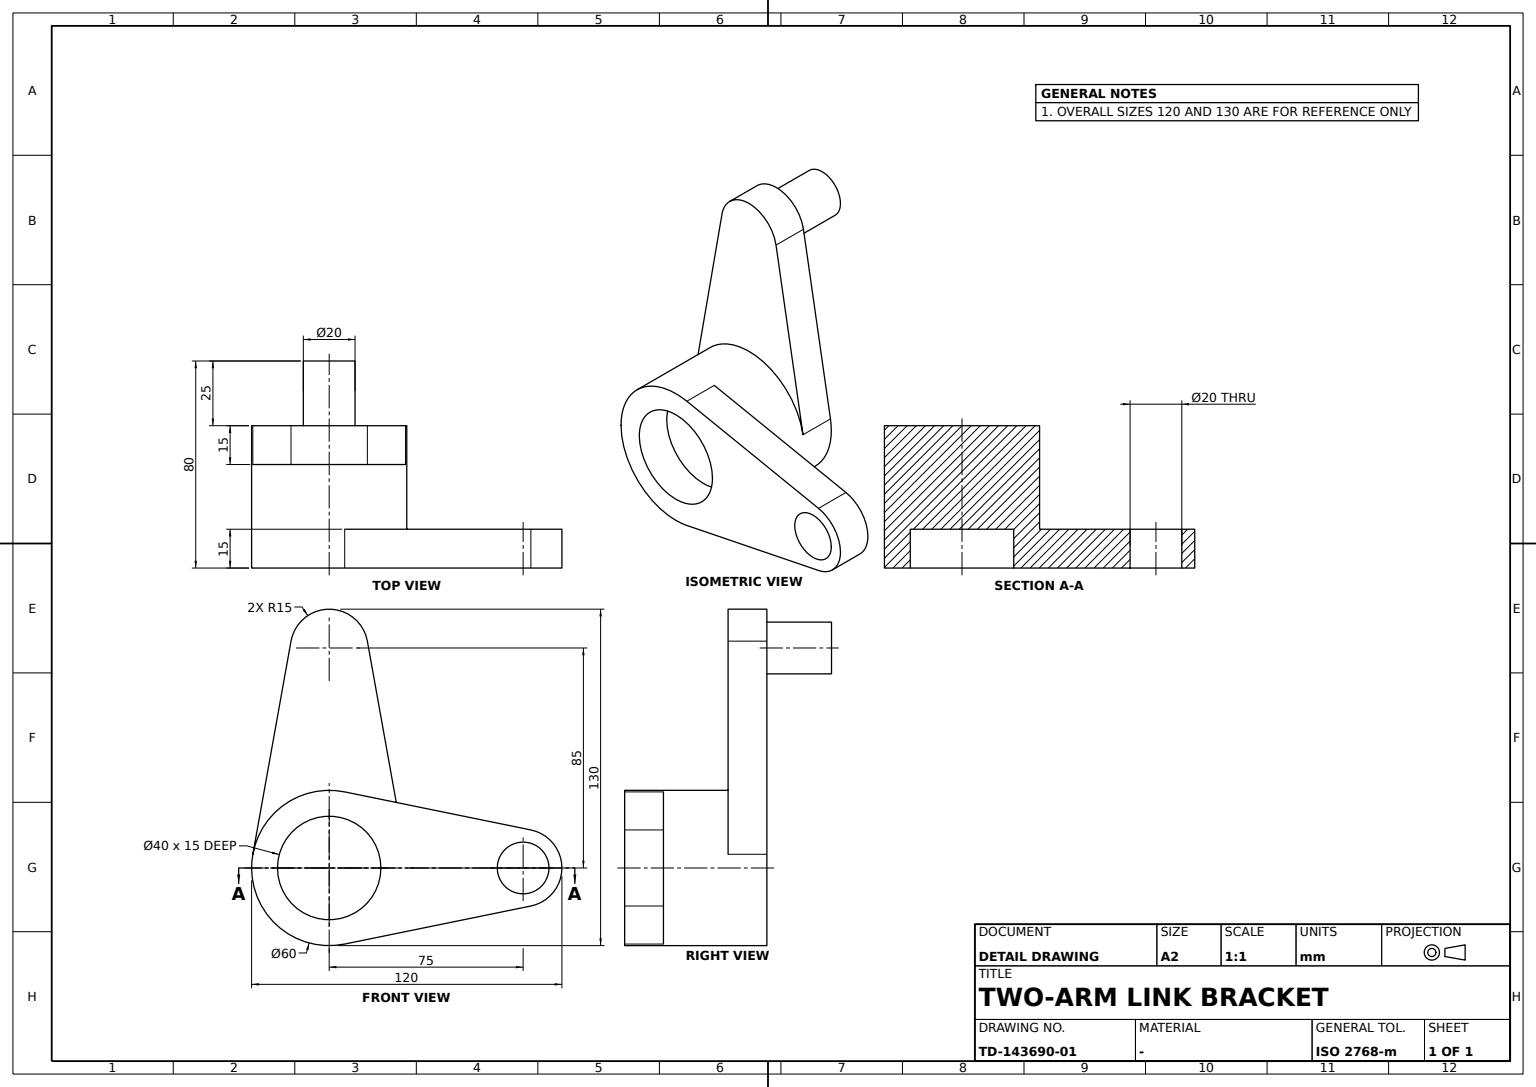
ISO-10303-21;
HEADER;
FILE_DESCRIPTION((''),'2;1');
FILE_NAME('','',(''),(''),'','','');
FILE_SCHEMA(('AUTOMOTIVE_DESIGN'));
ENDSEC;
DATA;
#1=APPLICATION_CONTEXT('');
#2=PRODUCT_CONTEXT('',#1,'mechanical');
#3=PRODUCT('','','',(#2));
#4=PRODUCT_DEFINITION_FORMATION('','',#3);
#5=PRODUCT_DEFINITION_CONTEXT('',#1,'design');
#6=PRODUCT_DEFINITION('','',#4,#5);
#7=PRODUCT_DEFINITION_SHAPE('','',#6);
#8=(LENGTH_UNIT()NAMED_UNIT(*)SI_UNIT(.MILLI.,.METRE.));
#9=(NAMED_UNIT(*)PLANE_ANGLE_UNIT()SI_UNIT($,.RADIAN.));
#10=(NAMED_UNIT(*)SI_UNIT($,.STERADIAN.)SOLID_ANGLE_UNIT());
#11=UNCERTAINTY_MEASURE_WITH_UNIT(LENGTH_MEASURE(1.E-05),#8,'distance_accuracy_value','');
#12=(GEOMETRIC_REPRESENTATION_CONTEXT(3)GLOBAL_UNCERTAINTY_ASSIGNED_CONTEXT((#11))GLOBAL_UNIT_ASSIGNED_CONTEXT((#8,#9,#10))REPRESENTATION_CONTEXT('',''));
#13=CARTESIAN_POINT('',(40.,85.,0.));
#14=VERTEX_POINT('',#13);
#15=CARTESIAN_POINT('',(40.,65.,0.));
#16=VERTEX_POINT('',#15);
#17=CARTESIAN_POINT('',(40.,75.,0.));
#18=DIRECTION('',(1.,0.,0.));
#19=DIRECTION('',(0.,1.,0.));
#20=AXIS2_PLACEMENT_3D('',#17,#18,#19);
#21=CIRCLE('',#20,10.);
#22=EDGE_CURVE('',#14,#16,#21,.T.);
#23=ORIENTED_EDGE('',*,*,#22,.F.);
#24=CARTESIAN_POINT('',(55.,85.,0.));
#25=VERTEX_POINT('',#24);
#26=CARTESIAN_POINT('',(47.5,85.,0.));
#27=DIRECTION('',(-1.,0.,0.));
#28=VECTOR('',#27,1000.);
#29=LINE('',#26,#28);
#30=EDGE_CURVE('',#25,#14,#29,.T.);
#31=ORIENTED_EDGE('',*,*,#30,.F.);
#32=CARTESIAN_POINT('',(55.,65.,0.));
#33=VERTEX_POINT('',#32);
#34=CARTESIAN_POINT('',(55.,75.,0.));
#35=AXIS2_PLACEMENT_3D('',#34,#18,#19);
#36=CIRCLE('',#35,10.);
#37=EDGE_CURVE('',#25,#33,#36,.T.);
#38=ORIENTED_EDGE('',*,*,#37,.T.);
#39=CARTESIAN_POINT('',(47.5,65.,0.));
#40=LINE('',#39,#28);
#41=EDGE_CURVE('',#33,#16,#40,.T.);
#42=ORIENTED_EDGE('',*,*,#41,.T.);
#43=EDGE_LOOP('',(#23,#31,#38,#42));
#44=FACE_OUTER_BOUND('',#43,.T.);
#45=CARTESIAN_POINT('',(47.5,75.,0.));
#46=AXIS2_PLACEMENT_3D('',#45,#27,#19);
#47=CYLINDRICAL_SURFACE('',#46,10.);
#48=ADVANCED_FACE('',(#44),#47,.F.);
#49=CARTESIAN_POINT('',(0.,-10.,85.));
#50=VERTEX_POINT('',#49);
#51=CARTESIAN_POINT('',(0.,10.,85.));
#52=VERTEX_POINT('',#51);
#53=CARTESIAN_POINT('',(0.,0.,85.));
#54=DIRECTION('',(0.,-1.,0.));
#55=AXIS2_PLACEMENT_3D('',#53,#27,#54);
#56=CIRCLE('',#55,10.);
#57=EDGE_CURVE('',#50,#52,#56,.T.);
#58=ORIENTED_EDGE('',*,*,#57,.F.);
#59=EDGE_CURVE('',#52,#50,#56,.T.);
#60=ORIENTED_EDGE('',*,*,#59,.F.);
#61=EDGE_LOOP('',(#58,#60));
#62=FACE_BOUND('',#61,.T.);
#63=CARTESIAN_POINT('',(0.,-14.764587,87.64707));
#64=VERTEX_POINT('',#63);
#65=CARTESIAN_POINT('',(0.,-29.529175,5.294128));
#66=VERTEX_POINT('',#65);
#67=CARTESIAN_POINT('',(0.,-22.146881,46.470599));
#68=DIRECTION('',(0.,-0.176470588,-0.984305914));
#69=VECTOR('',#68,1000.);
#70=LINE('',#67,#69);
#71=EDGE_CURVE('',#64,#66,#70,.T.);
#72=ORIENTED_EDGE('',*,*,#71,.F.);
#73=CARTESIAN_POINT('',(0.,14.764589,87.647059));
#74=VERTEX_POINT('',#73);
#75=AXIS2_PLACEMENT_3D('',#53,#18,#19);
#76=CIRCLE('',#75,15.);
#77=EDGE_CURVE('',#74,#64,#76,.T.);
#78=ORIENTED_EDGE('',*,*,#77,.F.);
#79=CARTESIAN_POINT('',(0.,29.529177,5.294118));
#80=VERTEX_POINT('',#79);
#81=CARTESIAN_POINT('',(0.,22.146883,46.470588));
#82=DIRECTION('',(0.,0.176470588,-0.984305914));
#83=VECTOR('',#82,1000.);
#84=LINE('',#81,#83);
#85=EDGE_CURVE('',#74,#80,#84,.T.);
#86=ORIENTED_EDGE('',*,*,#85,.T.);
#87=CARTESIAN_POINT('',(0.,30.,0.));
#88=VERTEX_POINT('',#87);
#89=CARTESIAN_POINT('',(0.,0.,0.));
#90=AXIS2_PLACEMENT_3D('',#89,#18,#19);
#91=CIRCLE('',#90,30.);
#92=EDGE_CURVE('',#88,#80,#91,.T.);
#93=ORIENTED_EDGE('',*,*,#92,.F.);
#94=CARTESIAN_POINT('',(0.,-30.,0.));
#95=VERTEX_POINT('',#94);
#96=EDGE_CURVE('',#95,#88,#91,.T.);
#97=ORIENTED_EDGE('',*,*,#96,.F.);
#98=EDGE_CURVE('',#66,#95,#91,.T.);
#99=ORIENTED_EDGE('',*,*,#98,.F.);
#100=EDGE_LOOP('',(#72,#78,#86,#93,#97,#99));
#101=FACE_OUTER_BOUND('',#100,.T.);
#102=PLANE('',#90);
#103=ADVANCED_FACE('',(#62,#101),#102,.F.);
#104=EDGE_CURVE('',#33,#25,#36,.T.);
#105=ORIENTED_EDGE('',*,*,#104,.T.);
#106=ORIENTED_EDGE('',*,*,#30,.T.);
#107=EDGE_CURVE('',#16,#14,#21,.T.);
#108=ORIENTED_EDGE('',*,*,#107,.F.);
#109=ORIENTED_EDGE('',*,*,#41,.F.);
#110=EDGE_LOOP('',(#105,#106,#108,#109));
#111=FACE_OUTER_BOUND('',#110,.T.);
#112=ADVANCED_FACE('',(#111),#47,.F.);
#113=CARTESIAN_POINT('',(40.,78.,-14.696938));
#114=VERTEX_POINT('',#113);
#115=CARTESIAN_POINT('',(40.,90.,0.));
#116=VERTEX_POINT('',#115);
#117=CIRCLE('',#20,15.);
#118=EDGE_CURVE('',#114,#116,#117,.T.);
#119=ORIENTED_EDGE('',*,*,#118,.T.);
#120=CARTESIAN_POINT('',(55.,90.,0.));
#121=VERTEX_POINT('',#120);
#122=CARTESIAN_POINT('',(47.5,90.,0.));
#123=LINE('',#122,#28);
#124=EDGE_CURVE('',#121,#116,#123,.T.);
#125=ORIENTED_EDGE('',*,*,#124,.F.);
#126=CARTESIAN_POINT('',(55.,78.,-14.696938));
#127=VERTEX_POINT('',#126);
#128=CIRCLE('',#35,15.);
#129=EDGE_CURVE('',#127,#121,#128,.T.);
#130=ORIENTED_EDGE('',*,*,#129,.F.);
#131=CARTESIAN_POINT('',(47.5,78.,-14.696938));
#132=LINE('',#131,#28);
#133=EDGE_CURVE('',#127,#114,#132,.T.);
#134=ORIENTED_EDGE('',*,*,#133,.T.);
#135=EDGE_LOOP('',(#119,#125,#130,#134));
#136=FACE_OUTER_BOUND('',#135,.T.);
#137=CYLINDRICAL_SURFACE('',#46,15.);
#138=ADVANCED_FACE('',(#136),#137,.T.);
#139=CARTESIAN_POINT('',(-25.,10.,85.));
#140=VERTEX_POINT('',#139);
#141=CARTESIAN_POINT('',(-12.5,10.,85.));
#142=LINE('',#141,#28);
#143=EDGE_CURVE('',#52,#140,#142,.T.);
#144=ORIENTED_EDGE('',*,*,#143,.F.);
#145=ORIENTED_EDGE('',*,*,#59,.T.);
#146=CARTESIAN_POINT('',(-25.,-10.,85.));
#147=VERTEX_POINT('',#146);
#148=CARTESIAN_POINT('',(-12.5,-10.,85.));
#149=LINE('',#148,#28);
#150=EDGE_CURVE('',#50,#147,#149,.T.);
#151=ORIENTED_EDGE('',*,*,#150,.T.);
#152=CARTESIAN_POINT('',(-25.,0.,85.));
#153=AXIS2_PLACEMENT_3D('',#152,#27,#54);
#154=CIRCLE('',#153,10.);
#155=EDGE_CURVE('',#140,#147,#154,.T.);
#156=ORIENTED_EDGE('',*,*,#155,.F.);
#157=EDGE_LOOP('',(#144,#145,#151,#156));
#158=FACE_OUTER_BOUND('',#157,.T.);
#159=CARTESIAN_POINT('',(-12.5,0.,85.));
#160=AXIS2_PLACEMENT_3D('',#159,#18,#54);
#161=CYLINDRICAL_SURFACE('',#160,10.);
#162=ADVANCED_FACE('',(#158),#161,.T.);
#163=CARTESIAN_POINT('',(40.,78.,14.696938));
#164=VERTEX_POINT('',#163);
#165=CARTESIAN_POINT('',(40.,6.,29.393877));
#166=VERTEX_POINT('',#165);
#167=CARTESIAN_POINT('',(40.,42.,22.045408));
#168=DIRECTION('',(0.,-0.979795897,0.2));
#169=VECTOR('',#168,1000.);
#170=LINE('',#167,#169);
#171=EDGE_CURVE('',#164,#166,#170,.T.);
#172=ORIENTED_EDGE('',*,*,#171,.F.);
#173=EDGE_CURVE('',#116,#164,#117,.T.);
#174=ORIENTED_EDGE('',*,*,#173,.F.);
#175=ORIENTED_EDGE('',*,*,#118,.F.);
#176=CARTESIAN_POINT('',(40.,6.,-29.393877));
#177=VERTEX_POINT('',#176);
#178=CARTESIAN_POINT('',(40.,42.,-22.045408));
#179=DIRECTION('',(0.,0.979795897,0.2));
#180=VECTOR('',#179,1000.);
#181=LINE('',#178,#180);
#182=EDGE_CURVE('',#177,#114,#181,.T.);
#183=ORIENTED_EDGE('',*,*,#182,.F.);
#184=CARTESIAN_POINT('',(40.,30.,0.));
#185=VERTEX_POINT('',#184);
#186=CARTESIAN_POINT('',(40.,0.,0.));
#187=AXIS2_PLACEMENT_3D('',#186,#18,#19);
#188=CIRCLE('',#187,30.);
#189=EDGE_CURVE('',#177,#185,#188,.T.);
#190=ORIENTED_EDGE('',*,*,#189,.T.);
#191=CARTESIAN_POINT('',(40.,29.529177,5.294118));
#192=VERTEX_POINT('',#191);
#193=EDGE_CURVE('',#185,#192,#188,.T.);
#194=ORIENTED_EDGE('',*,*,#193,.T.);
#195=AXIS2_PLACEMENT_3D('',#186,#27,#19);
#196=CIRCLE('',#195,30.);
#197=EDGE_CURVE('',#166,#192,#196,.T.);
#198=ORIENTED_EDGE('',*,*,#197,.F.);
#199=EDGE_LOOP('',(#172,#174,#175,#183,#190,#194,#198));
#200=FACE_OUTER_BOUND('',#199,.T.);
#201=ORIENTED_EDGE('',*,*,#107,.T.);
#202=ORIENTED_EDGE('',*,*,#22,.T.);
#203=EDGE_LOOP('',(#201,#202));
#204=FACE_BOUND('',#203,.T.);
#205=PLANE('',#187);
#206=ADVANCED_FACE('',(#200,#204),#205,.F.);
#207=CARTESIAN_POINT('',(40.,-20.,0.));
#208=VERTEX_POINT('',#207);
#209=CARTESIAN_POINT('',(40.,20.,0.));
#210=VERTEX_POINT('',#209);
#211=CIRCLE('',#187,20.);
#212=EDGE_CURVE('',#208,#210,#211,.T.);
#213=ORIENTED_EDGE('',*,*,#212,.F.);
#214=CARTESIAN_POINT('',(55.,-20.,0.));
#215=VERTEX_POINT('',#214);
#216=CARTESIAN_POINT('',(47.5,-20.,0.));
#217=LINE('',#216,#28);
#218=EDGE_CURVE('',#215,#208,#217,.T.);
#219=ORIENTED_EDGE('',*,*,#218,.F.);
#220=CARTESIAN_POINT('',(55.,20.,0.));
#221=VERTEX_POINT('',#220);
#222=CARTESIAN_POINT('',(55.,0.,0.));
#223=AXIS2_PLACEMENT_3D('',#222,#18,#19);
#224=CIRCLE('',#223,20.);
#225=EDGE_CURVE('',#215,#221,#224,.T.);
#226=ORIENTED_EDGE('',*,*,#225,.T.);
#227=CARTESIAN_POINT('',(47.5,20.,0.));
#228=LINE('',#227,#28);
#229=EDGE_CURVE('',#221,#210,#228,.T.);
#230=ORIENTED_EDGE('',*,*,#229,.T.);
#231=EDGE_LOOP('',(#213,#219,#226,#230));
#232=FACE_OUTER_BOUND('',#231,.T.);
#233=CARTESIAN_POINT('',(47.5,0.,0.));
#234=AXIS2_PLACEMENT_3D('',#233,#27,#19);
#235=CYLINDRICAL_SURFACE('',#234,20.);
#236=ADVANCED_FACE('',(#232),#235,.F.);
#237=ORIENTED_EDGE('',*,*,#155,.T.);
#238=EDGE_CURVE('',#147,#140,#154,.T.);
#239=ORIENTED_EDGE('',*,*,#238,.T.);
#240=EDGE_LOOP('',(#237,#239));
#241=FACE_OUTER_BOUND('',#240,.T.);
#242=CARTESIAN_POINT('',(-25.,0.,0.));
#243=AXIS2_PLACEMENT_3D('',#242,#27,#54);
#244=PLANE('',#243);
#245=ADVANCED_FACE('',(#241),#244,.T.);
#246=ORIENTED_EDGE('',*,*,#193,.F.);
#247=CARTESIAN_POINT('',(27.5,30.,0.));
#248=LINE('',#247,#28);
#249=EDGE_CURVE('',#185,#88,#248,.T.);
#250=ORIENTED_EDGE('',*,*,#249,.T.);
#251=ORIENTED_EDGE('',*,*,#92,.T.);
#252=CARTESIAN_POINT('',(15.,29.529177,5.294118));
#253=VERTEX_POINT('',#252);
#254=CARTESIAN_POINT('',(7.5,29.529177,5.294118));
#255=VECTOR('',#18,1000.);
#256=LINE('',#254,#255);
#257=EDGE_CURVE('',#80,#253,#256,.T.);
#258=ORIENTED_EDGE('',*,*,#257,.T.);
#259=CARTESIAN_POINT('',(27.5,29.529177,5.294118));
#260=LINE('',#259,#255);
#261=EDGE_CURVE('',#253,#192,#260,.T.);
#262=ORIENTED_EDGE('',*,*,#261,.T.);
#263=EDGE_LOOP('',(#246,#250,#251,#258,#262));
#264=FACE_OUTER_BOUND('',#263,.T.);
#265=CARTESIAN_POINT('',(27.5,0.,0.));
#266=AXIS2_PLACEMENT_3D('',#265,#27,#19);
#267=CYLINDRICAL_SURFACE('',#266,30.);
#268=ADVANCED_FACE('',(#264),#267,.T.);
#269=CARTESIAN_POINT('',(15.,-29.529175,5.294128));
#270=VERTEX_POINT('',#269);
#271=CARTESIAN_POINT('',(55.,-29.529175,5.294128));
#272=VERTEX_POINT('',#271);
#273=CARTESIAN_POINT('',(27.5,-29.529175,5.294128));
#274=LINE('',#273,#255);
#275=EDGE_CURVE('',#270,#272,#274,.T.);
#276=ORIENTED_EDGE('',*,*,#275,.F.);
#277=CARTESIAN_POINT('',(7.5,-29.529175,5.294128));
#278=LINE('',#277,#255);
#279=EDGE_CURVE('',#66,#270,#278,.T.);
#280=ORIENTED_EDGE('',*,*,#279,.F.);
#281=ORIENTED_EDGE('',*,*,#98,.T.);
#282=CARTESIAN_POINT('',(55.,-30.,0.));
#283=VERTEX_POINT('',#282);
#284=CARTESIAN_POINT('',(27.5,-30.,0.));
#285=LINE('',#284,#28);
#286=EDGE_CURVE('',#283,#95,#285,.T.);
#287=ORIENTED_EDGE('',*,*,#286,.F.);
#288=CIRCLE('',#223,30.);
#289=EDGE_CURVE('',#272,#283,#288,.T.);
#290=ORIENTED_EDGE('',*,*,#289,.F.);
#291=EDGE_LOOP('',(#276,#280,#281,#287,#290));
#292=FACE_OUTER_BOUND('',#291,.T.);
#293=ADVANCED_FACE('',(#292),#267,.T.);
#294=CARTESIAN_POINT('',(15.,14.764589,87.647059));
#295=VERTEX_POINT('',#294);
#296=CARTESIAN_POINT('',(7.5,14.764589,87.647059));
#297=LINE('',#296,#255);
#298=EDGE_CURVE('',#74,#295,#297,.T.);
#299=ORIENTED_EDGE('',*,*,#298,.T.);
#300=CARTESIAN_POINT('',(15.,22.146883,46.470588));
#301=LINE('',#300,#83);
#302=EDGE_CURVE('',#295,#253,#301,.T.);
#303=ORIENTED_EDGE('',*,*,#302,.T.);
#304=ORIENTED_EDGE('',*,*,#257,.F.);
#305=ORIENTED_EDGE('',*,*,#85,.F.);
#306=EDGE_LOOP('',(#299,#303,#304,#305));
#307=FACE_OUTER_BOUND('',#306,.T.);
#308=DIRECTION('',(0.,-0.984305914,-0.176470588));
#309=AXIS2_PLACEMENT_3D('',#73,#308,#82);
#310=PLANE('',#309);
#311=ADVANCED_FACE('',(#307),#310,.F.);
#312=CARTESIAN_POINT('',(55.,78.,14.696938));
#313=VERTEX_POINT('',#312);
#314=CARTESIAN_POINT('',(47.5,78.,14.696938));
#315=LINE('',#314,#28);
#316=EDGE_CURVE('',#313,#164,#315,.T.);
#317=ORIENTED_EDGE('',*,*,#316,.F.);
#318=EDGE_CURVE('',#121,#313,#128,.T.);
#319=ORIENTED_EDGE('',*,*,#318,.F.);
#320=ORIENTED_EDGE('',*,*,#124,.T.);
#321=ORIENTED_EDGE('',*,*,#173,.T.);
#322=EDGE_LOOP('',(#317,#319,#320,#321));
#323=FACE_OUTER_BOUND('',#322,.T.);
#324=ADVANCED_FACE('',(#323),#137,.T.);
#325=ORIENTED_EDGE('',*,*,#302,.F.);
#326=CARTESIAN_POINT('',(15.,-14.764587,87.64707));
#327=VERTEX_POINT('',#326);
#328=CARTESIAN_POINT('',(15.,0.,85.));
#329=AXIS2_PLACEMENT_3D('',#328,#18,#19);
#330=CIRCLE('',#329,15.);
#331=EDGE_CURVE('',#295,#327,#330,.T.);
#332=ORIENTED_EDGE('',*,*,#331,.T.);
#333=CARTESIAN_POINT('',(15.,-22.146881,46.470599));
#334=LINE('',#333,#69);
#335=EDGE_CURVE('',#327,#270,#334,.T.);
#336=ORIENTED_EDGE('',*,*,#335,.T.);
#337=CARTESIAN_POINT('',(15.,0.,0.));
#338=AXIS2_PLACEMENT_3D('',#337,#18,#19);
#339=CIRCLE('',#338,30.);
#340=EDGE_CURVE('',#253,#270,#339,.T.);
#341=ORIENTED_EDGE('',*,*,#340,.F.);
#342=EDGE_LOOP('',(#325,#332,#336,#341));
#343=FACE_OUTER_BOUND('',#342,.T.);
#344=PLANE('',#338);
#345=ADVANCED_FACE('',(#343),#344,.T.);
#346=ORIENTED_EDGE('',*,*,#275,.T.);
#347=CARTESIAN_POINT('',(55.,6.,29.393877));
#348=VERTEX_POINT('',#347);
#349=EDGE_CURVE('',#348,#272,#288,.T.);
#350=ORIENTED_EDGE('',*,*,#349,.F.);
#351=CARTESIAN_POINT('',(27.5,6.,29.393877));
#352=LINE('',#351,#28);
#353=EDGE_CURVE('',#348,#166,#352,.T.);
#354=ORIENTED_EDGE('',*,*,#353,.T.);
#355=ORIENTED_EDGE('',*,*,#197,.T.);
#356=ORIENTED_EDGE('',*,*,#261,.F.);
#357=ORIENTED_EDGE('',*,*,#340,.T.);
#358=EDGE_LOOP('',(#346,#350,#354,#355,#356,#357));
#359=FACE_OUTER_BOUND('',#358,.T.);
#360=ADVANCED_FACE('',(#359),#267,.T.);
#361=ORIENTED_EDGE('',*,*,#335,.F.);
#362=CARTESIAN_POINT('',(7.5,-14.764587,87.64707));
#363=LINE('',#362,#255);
#364=EDGE_CURVE('',#64,#327,#363,.T.);
#365=ORIENTED_EDGE('',*,*,#364,.F.);
#366=ORIENTED_EDGE('',*,*,#71,.T.);
#367=ORIENTED_EDGE('',*,*,#279,.T.);
#368=EDGE_LOOP('',(#361,#365,#366,#367));
#369=FACE_OUTER_BOUND('',#368,.T.);
#370=DIRECTION('',(0.,-0.984305914,0.176470588));
#371=AXIS2_PLACEMENT_3D('',#63,#370,#68);
#372=PLANE('',#371);
#373=ADVANCED_FACE('',(#369),#372,.T.);
#374=ORIENTED_EDGE('',*,*,#150,.F.);
#375=ORIENTED_EDGE('',*,*,#57,.T.);
#376=ORIENTED_EDGE('',*,*,#143,.T.);
#377=ORIENTED_EDGE('',*,*,#238,.F.);
#378=EDGE_LOOP('',(#374,#375,#376,#377));
#379=FACE_OUTER_BOUND('',#378,.T.);
#380=ADVANCED_FACE('',(#379),#161,.T.);
#381=ORIENTED_EDGE('',*,*,#212,.T.);
#382=EDGE_CURVE('',#210,#208,#211,.T.);
#383=ORIENTED_EDGE('',*,*,#382,.T.);
#384=EDGE_LOOP('',(#381,#383));
#385=FACE_OUTER_BOUND('',#384,.T.);
#386=ADVANCED_FACE('',(#385),#205,.T.);
#387=EDGE_CURVE('',#221,#215,#224,.T.);
#388=ORIENTED_EDGE('',*,*,#387,.T.);
#389=ORIENTED_EDGE('',*,*,#218,.T.);
#390=ORIENTED_EDGE('',*,*,#382,.F.);
#391=ORIENTED_EDGE('',*,*,#229,.F.);
#392=EDGE_LOOP('',(#388,#389,#390,#391));
#393=FACE_OUTER_BOUND('',#392,.T.);
#394=ADVANCED_FACE('',(#393),#235,.F.);
#395=ORIENTED_EDGE('',*,*,#298,.F.);
#396=ORIENTED_EDGE('',*,*,#77,.T.);
#397=ORIENTED_EDGE('',*,*,#364,.T.);
#398=ORIENTED_EDGE('',*,*,#331,.F.);
#399=EDGE_LOOP('',(#395,#396,#397,#398));
#400=FACE_OUTER_BOUND('',#399,.T.);
#401=CARTESIAN_POINT('',(7.5,0.,85.));
#402=AXIS2_PLACEMENT_3D('',#401,#27,#19);
#403=CYLINDRICAL_SURFACE('',#402,15.);
#404=ADVANCED_FACE('',(#400),#403,.T.);
#405=ORIENTED_EDGE('',*,*,#133,.F.);
#406=CARTESIAN_POINT('',(55.,6.,-29.393877));
#407=VERTEX_POINT('',#406);
#408=CARTESIAN_POINT('',(55.,42.,-22.045408));
#409=LINE('',#408,#180);
#410=EDGE_CURVE('',#407,#127,#409,.T.);
#411=ORIENTED_EDGE('',*,*,#410,.F.);
#412=CARTESIAN_POINT('',(27.5,6.,-29.393877));
#413=LINE('',#412,#255);
#414=EDGE_CURVE('',#177,#407,#413,.T.);
#415=ORIENTED_EDGE('',*,*,#414,.F.);
#416=ORIENTED_EDGE('',*,*,#182,.T.);
#417=EDGE_LOOP('',(#405,#411,#415,#416));
#418=FACE_OUTER_BOUND('',#417,.T.);
#419=DIRECTION('',(0.,-0.2,0.979795897));
#420=AXIS2_PLACEMENT_3D('',#406,#419,#179);
#421=PLANE('',#420);
#422=ADVANCED_FACE('',(#418),#421,.F.);
#423=ORIENTED_EDGE('',*,*,#171,.T.);
#424=ORIENTED_EDGE('',*,*,#353,.F.);
#425=CARTESIAN_POINT('',(55.,42.,22.045408));
#426=LINE('',#425,#169);
#427=EDGE_CURVE('',#313,#348,#426,.T.);
#428=ORIENTED_EDGE('',*,*,#427,.F.);
#429=ORIENTED_EDGE('',*,*,#316,.T.);
#430=EDGE_LOOP('',(#423,#424,#428,#429));
#431=FACE_OUTER_BOUND('',#430,.T.);
#432=DIRECTION('',(0.,0.2,0.979795897));
#433=DIRECTION('',(0.,0.979795897,-0.2));
#434=AXIS2_PLACEMENT_3D('',#347,#432,#433);
#435=PLANE('',#434);
#436=ADVANCED_FACE('',(#431),#435,.T.);
#437=ORIENTED_EDGE('',*,*,#189,.F.);
#438=ORIENTED_EDGE('',*,*,#414,.T.);
#439=EDGE_CURVE('',#283,#407,#288,.T.);
#440=ORIENTED_EDGE('',*,*,#439,.F.);
#441=ORIENTED_EDGE('',*,*,#286,.T.);
#442=ORIENTED_EDGE('',*,*,#96,.T.);
#443=ORIENTED_EDGE('',*,*,#249,.F.);
#444=EDGE_LOOP('',(#437,#438,#440,#441,#442,#443));
#445=FACE_OUTER_BOUND('',#444,.T.);
#446=ADVANCED_FACE('',(#445),#267,.T.);
#447=ORIENTED_EDGE('',*,*,#225,.F.);
#448=ORIENTED_EDGE('',*,*,#387,.F.);
#449=EDGE_LOOP('',(#447,#448));
#450=FACE_BOUND('',#449,.T.);
#451=ORIENTED_EDGE('',*,*,#37,.F.);
#452=ORIENTED_EDGE('',*,*,#104,.F.);
#453=EDGE_LOOP('',(#451,#452));
#454=FACE_BOUND('',#453,.T.);
#455=ORIENTED_EDGE('',*,*,#129,.T.);
#456=ORIENTED_EDGE('',*,*,#318,.T.);
#457=ORIENTED_EDGE('',*,*,#427,.T.);
#458=ORIENTED_EDGE('',*,*,#349,.T.);
#459=ORIENTED_EDGE('',*,*,#289,.T.);
#460=ORIENTED_EDGE('',*,*,#439,.T.);
#461=ORIENTED_EDGE('',*,*,#410,.T.);
#462=EDGE_LOOP('',(#455,#456,#457,#458,#459,#460,#461));
#463=FACE_OUTER_BOUND('',#462,.T.);
#464=PLANE('',#223);
#465=ADVANCED_FACE('',(#450,#454,#463),#464,.T.);
#466=CLOSED_SHELL('',(#48,#103,#112,#138,#162,#206,#236,#245,#268,#293,#311,#324,#345,#360,#373,#380,#386,#394,#404,#422,#436,#446,#465));
#467=MANIFOLD_SOLID_BREP('',#466);
#468=ADVANCED_BREP_SHAPE_REPRESENTATION('',(#467),#12);
#469=SHAPE_DEFINITION_REPRESENTATION(#7,#468);
ENDSEC;
END-ISO-10303-21;
